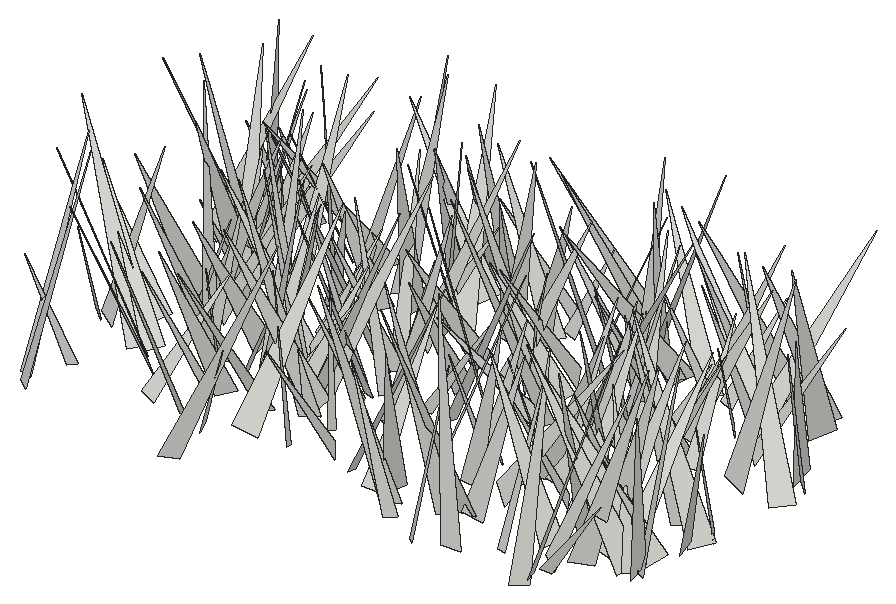
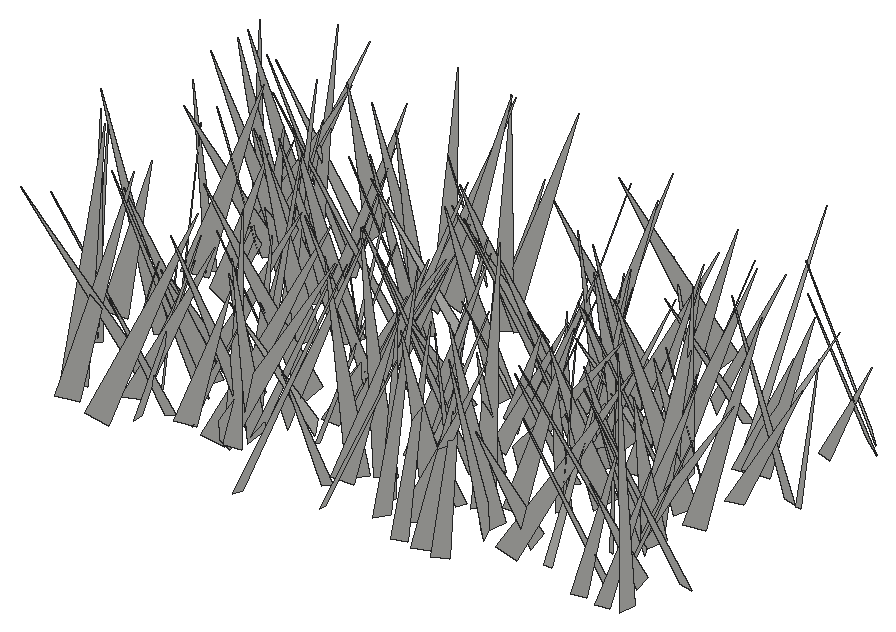
# SketchUp Ruby script. Lengths in inches.
U = 1.inch
M = Sketchup.active_model
def pt(a) = Geom::Point3d.new(a.map { |v| v * U })
def face(e, loops, mat)
  f = e.add_face(loops[0].map { |a| pt(a) })
  loops[1..].each { |l| e.add_face(l.map { |a| pt(a) }).erase! }
  f.material = f.back_material = mat if mat
  f
end
# faces: each face lists its corners as indices into pts; further lists are holes
def faces(e, pts, list, mat = nil) = list.each { |f| face(e, (f[0].is_a?(Array) ? f : [f]).map { |l| l.map { |i| pts[i] } }, mat) }
# xy, xz, yz: faces in a plane at the given z, y or x. An outline is a flat list of corners, or four numbers for a rectangle; further outlines are holes
def ring(l) = l.size == 4 ? [[l[0], l[1]], [l[2], l[1]], [l[2], l[3]], [l[0], l[3]]] : l.each_slice(2).to_a
def flat(e, list, mat, &to3) = list.each { |f| face(e, (f[0].is_a?(Array) ? f : [f]).map { |l| ring(l).map { |u, v| to3.(u, v) } }, mat) }
def xy(e, z, list, mat = nil) = flat(e, list, mat) { |x, y| [x, y, z] }
def xz(e, y, list, mat = nil) = flat(e, list, mat) { |x, z| [x, y, z] }
def yz(e, x, list, mat = nil) = flat(e, list, mat) { |y, z| [x, y, z] }
def lines(e, pts, list) = list.each { |a, b| e.add_line(pt(pts[a]), pt(pts[b])) }
# prism: a flat outline (further loops are holes) pulled along v
def prism(e, loops, v, mat = nil)
  f = face(e, loops, mat); d = Geom::Vector3d.new(v.map { |x| x * U })
  f.pushpull(f.normal.samedirection?(d) ? d.length : -d.length)
end
def box(e, o, s, mat = nil) = prism(e, [[o, [o[0] + s[0], o[1], o[2]], [o[0] + s[0], o[1] + s[1], o[2]], [o[0], o[1] + s[1], o[2]]]], [0, 0, s[2]], mat)
def at(x, y, z, deg = 0) = Geom::Transformation.translation(pt([x, y, z])) * Geom::Transformation.rotation(ORIGIN, Z_AXIS, deg.degrees)
def axes(o, x, y, z) = Geom::Transformation.new([*x, 0, *y, 0, *z, 0, *pt(o).to_a, 1])
def part(name) = M.definitions.add(name)
# library, detail: a bought-in or finely detailed component or shape, given as its bounding box
def library(name, o, s) = part(name).tap { |d| box(d.entities, o, s) }
def detail(e, o, s) = box(e.add_group.entities, o, s)
def put(e, d, t, mat = nil) = e.add_instance(d, t).tap { |i| i.material = mat if mat }
def group(e, t, mat = nil) = e.add_group.tap { |g| g.transformation = t; g.material = mat if mat }.entities
root = M.entities
c1 = part("fur_instance\#9")
p = [[0.8125,0,1.79],[0.67,-0.02,1.48],[0,-0.11,0],[0,0.11,0]]
faces(c1.entities,p,[[0,1,2,3]])
put(root,c1,axes([530.97,285.85,-21.66],[-1.13244,4.66111,1.93868],[4.91983,0.57378,1.4943],[-1.13125,-2.17064,4.55801]))
put(root,c1,axes([515.75,283.15,-21.66],[7.47799,-1.52657,1.95795],[-2.25093,-6.79047,3.30259],[-1.04752,3.69369,6.88067]))
put(root,c1,axes([529.06,288.6,-21.66],[6.38115,-3.67921,0.2036],[-3.55943,-6.25987,-1.56256],[-0.95316,-1.25481,7.1982]))
put(root,c1,axes([536.32,285.05,-21.66],[0.66704,7.88186,2.68055],[8.14998,-1.16705,1.40349],[-1.69907,-2.50365,7.78452]))
put(root,c1,axes([529.87,287.22,-21.66],[-0.48012,-7.554,2.16495],[-7.6037,-0.10085,-2.03814],[-1.98335,2.21526,7.28968]))
put(root,c1,axes([533.84,284.27,-21.66],[3.8094,4.08661,1.06154],[3.80016,-3.94157,1.53675],[-1.84012,0.32005,5.37125]))
put(root,c1,axes([515.07,287.34,-21.66],[4.19489,0.81761,0.41517],[0.91291,-3.90671,-1.53042],[-0.08632,-1.58339,3.99042]))
put(root,c1,axes([542.66,286.41,-21.66],[2.65844,-2.5721,0.0216],[-2.2994,-2.3625,1.67773],[1.15278,1.21916,3.2967]))
put(root,c1,axes([523.16,290.16,-21.66],[-4.76497,-3.93422,0.44703],[-3.2824,4.31602,2.99679],[2.21445,-2.06803,5.40391]))
put(root,c1,axes([542.42,284.16,-21.66],[-6.84761,2.51212,1.52779],[1.98246,6.80446,-2.30302],[2.17135,1.70976,6.92074]))
put(root,c1,axes([534.45,288.99,-21.66],[-1.86183,-7.54983,1.10161],[-7.50699,1.61006,-1.65309],[-1.3633,1.44488,7.59827]))
put(root,c1,axes([503.11,284.7,-21.66],[5.00071,5.94343,0.88428],[5.7504,-5.06729,1.53914],[-1.74336,0.3341,7.61331]))
put(root,c1,axes([533.54,288.07,-21.66],[-0.98581,-7.65367,2.64082],[-7.9173,0.35473,-1.92744],[-1.69382,2.79641,7.47232]))
put(root,c1,axes([513.05,287.875,-21.66],[-3.40667,-4.88664,0.79026],[-4.79108,3.01371,-2.01797],[-1.2447,1.77411,5.60468]))
put(root,c1,axes([507.74,291.31,-21.66],[-4.53794,-6.8341,0.16977],[-6.57814,4.42074,2.12406],[1.86058,-1.03861,7.92377]))
put(root,c1,axes([547.21,289.82,-21.66],[7.02659,-0.33713,1.59],[0.09653,-6.95626,-1.90152],[-1.62247,-1.87389,6.7728]))
put(root,c1,axes([542.24,287.38,-21.66],[3.65176,6.04586,1.11201],[6.02251,-3.25936,-2.05677],[1.23222,-1.98709,6.75703]))
put(root,c1,axes([503.86,288.52,-21.66],[-0.24742,-3.68689,1.2628],[-3.55064,-0.30834,-1.59591],[-1.60648,1.24932,3.33279]))
put(root,c1,axes([542.32,285.37,-21.66],[7.12213,3.78972,1.00867],[3.4176,-7.02352,2.25704],[-1.92338,1.55314,7.74548]))
put(root,c1,axes([546.34,289.97,-21.66],[-7.92246,2.32052,1.49756],[2.68865,7.5204,2.57051],[0.63138,-2.90715,7.84491]))
put(root,c1,axes([542.16,291.02,-21.66],[-1.3783,-7.92591,0.91068],[-7.76861,1.54372,1.6777],[1.81604,0.58822,7.86798]))
put(root,c1,axes([512.99,290.77,-21.66],[-4.86193,-2.9811,0.43497],[-2.74592,4.72474,1.68858],[1.2394,-1.22654,5.44739]))
put(root,c1,axes([540.83,289.375,-21.66],[-5.87282,3.13064,1.60123],[3.47052,5.66214,1.65846],[0.56601,-2.23474,6.44519]))
put(root,c1,axes([513.48,291.58,-21.66],[3.27903,-5.74844,0.73311],[-5.41958,-3.34021,-1.9507],[-2.05188,-0.36394,6.32387]))
put(root,c1,axes([534.95,288.9,-21.66],[-0.35143,6.05342,2.99786],[6.31844,1.35633,-1.99808],[2.38924,-2.69649,5.72495]))
put(root,c1,axes([543.76,288.49,-21.66],[6.10397,-4.61293,1.81963],[-4.95361,-5.80478,1.9013],[-0.22786,2.62185,7.41098]))
put(root,c1,axes([502.4,285.78,-21.66],[3.79972,6.90357,0.39781],[6.61789,-3.76205,2.07507],[-2.00527,0.66563,7.60206]))
put(root,c1,axes([516.72,291.52,-21.66],[0.00181,-5.98408,0.19016],[-5.68264,-0.06159,-1.88392],[-1.88493,0.17992,5.67979]))
put(root,c1,axes([538.9,286.78,-21.66],[2.7978,5.22834,0.27095],[4.99402,-2.75746,1.64099],[-1.57121,0.54549,5.69828]))
put(root,c1,axes([547.18,291.66,-21.66],[-6.27712,3.42033,1.55819],[3.73626,5.34865,3.31076],[-0.40863,-3.63622,6.33559]))
put(root,c1,axes([510.05,288.2,-21.66],[1.05381,5.0713,0.10966],[4.76326,-0.95083,-1.80217],[1.74396,-0.4674,4.856]))
put(root,c1,axes([527.99,287.75,-21.66],[-2.51338,5.74575,1.01303],[5.46798,2.70448,-1.77311],[2.03497,-0.17044,6.01555]))
put(root,c1,axes([520.58,288.82,-21.66],[-5.03149,-1.83162,1.20846],[-2.18082,4.50919,-2.24552],[0.24343,2.5384,4.86091]))
put(root,c1,axes([519.12,293.67,-21.66],[-7.73279,0.49202,2.83462],[1.75633,7.24586,3.53356],[2.27869,-3.91518,6.89581]))
put(root,c1,axes([546.6875,292.45,-21.66],[-4.22388,-0.55824,1.0602],[-0.01996,3.91714,1.98304],[1.19803,-1.90295,3.77099]))
put(root,c1,axes([543.84,290.95,-21.66],[4.37755,-6.1842,1.75356],[-6.40379,-4.01166,1.83857],[0.55746,2.47882,7.3503]))
put(root,c1,axes([546.74,289.47,-21.66],[-0.83276,5.81039,0.96307],[5.68734,0.54058,1.65638],[-1.53047,-1.15272,5.63121]))
put(root,c1,axes([532.32,292.05,-21.66],[1.87666,-6.19619,1.68038],[-6.32701,-1.4881,1.57887],[1.08876,2.03251,6.27868]))
put(root,c1,axes([517.32,288.61,-21.66],[-1.94232,7.80928,1.11049],[7.41359,2.19794,-2.48968],[2.69386,-0.41817,7.65238]))
put(root,c1,axes([525.49,288.91,-21.66],[6.20269,2.14266,0.41588],[1.88774,-5.89525,2.21806],[-1.09562,1.97291,6.17613]))
put(root,c1,axes([538.27,294.13,-21.66],[-4.62318,-3.47557,0.41553],[-3.19467,4.47097,1.85217],[1.4305,-1.24775,5.47931]))
put(root,c1,axes([544.24,290.26,-21.66],[-0.17327,7.80384,1.95788],[7.72096,0.71202,-2.15474],[2.26272,-1.83203,7.50246]))
put(root,c1,axes([519.29,292.49,-21.66],[-0.93338,-7.69941,2.7531],[-7.87622,0.10215,-2.38461],[-2.19672,2.90522,7.38009]))
put(root,c1,axes([547.47,289.7,-21.66],[3.93388,5.26717,1.14139],[4.90502,-4.08461,1.94372],[-2.23307,0.30691,6.28017]))
put(root,c1,axes([542.2,294.74,-21.66],[-5.45284,-1.57742,1.94379],[-0.6971,5.43147,2.45217],[2.40429,-2.00271,5.11943]))
put(root,c1,axes([506.74,292.28,-21.66],[-5.49378,-4.48735,0.1731],[-4.21573,5.05933,-2.64174],[-1.54724,2.14821,6.58325]))
put(root,c1,axes([547.57,293.93,-21.66],[5.98567,0.36805,0.66862],[0.55714,-5.71998,-1.83907],[-0.52163,-1.88604,5.70802]))
put(root,c1,axes([534.47,292.25,-21.66],[4.68753,6.76488,0.69054],[6.04009,-3.75687,-4.19721],[3.12373,-2.88717,7.07954]))
put(root,c1,axes([510.81,294.57,-21.66],[0.32689,-6.93131,1.01824],[-6.72809,-0.59471,-1.88835],[-1.95261,0.88881,6.67713]))
put(root,c1,axes([501.14,294.5,-21.66],[-2.16154,-4.08693,0.6496],[-3.73051,2.24163,1.68984],[1.79115,-0.26331,4.30345]))
put(root,c1,axes([510.66,294.32,-21.66],[-2.98653,-2.99705,1.42564],[-2.58075,3.30304,1.53746],[2.08674,-0.20437,3.94181]))
put(root,c1,axes([532.27,292.78,-21.66],[0.67083,5.9533,2.27987],[6.17356,-0.03505,-1.72498],[1.58958,-2.37626,5.73727]))
put(root,c1,axes([545.71,290.08,-21.66],[-2.00066,7.03095,0.19663],[6.73059,1.97306,-2.06922],[2.04255,0.38513,7.01108]))
put(root,c1,axes([521.4,292.02,-21.66],[-4.31752,-0.25034,0.73123],[-0.52227,4.00392,-1.71296],[0.56974,1.77322,3.97108]))
put(root,c1,axes([539.76,296.52,-21.66],[-3.16207,-7.07316,1.24758],[-6.76016,3.39142,2.09364],[2.42619,0.2311,7.45956]))
put(root,c1,axes([530.11,291.04,-21.66],[5.9455,4.2001,0.21568],[4.05072,-5.81939,1.66213],[-1.13095,1.23699,7.08711]))
put(root,c1,axes([515.97,291.76,-21.66],[6.62272,2.03005,2.53711],[1.31072,-6.93962,2.13125],[-2.97322,1.46257,6.59085]))
put(root,c1,axes([520.82,295.73,-21.66],[-4.32918,-1.79601,0.73607],[-1.48596,4.22424,1.56749],[1.24875,-1.19977,4.41706]))
put(root,c1,axes([506.58,293.13,-21.66],[-3.94655,4.7323,0.06828],[4.56087,3.77904,1.70056],[-1.26405,-1.13963,5.92267]))
put(root,c1,axes([505.78,292.89,-21.66],[-4.22364,6.9226,0.63988],[6.72709,3.88063,2.42031],[-1.75445,-1.78585,7.73974]))
put(root,c1,axes([511.64,297.58,-21.66],[6.11084,-2.63091,1.80363],[-1.49433,-5.80472,-3.40432],[-2.81811,-2.62692,5.71618]))
put(root,c1,axes([532.14,294.27,-21.66],[-1.49858,-3.44059,1.04989],[-3.40031,0.98374,-1.62968],[-1.17382,1.54281,3.38047]))
put(root,c1,axes([501.99,294.28,-21.66],[3.4737,5.90005,1.74495],[6.11319,-3.08303,-1.74525],[0.69596,-2.36778,6.62052]))
put(root,c1,axes([548,296.24,-21.66],[-3.52584,-3.38703,1.52089],[-2.9555,3.82986,1.67745],[2.24724,-0.27722,4.59235]))
put(root,c1,axes([548.17,294.86,-21.66],[-5.06971,5.94983,1.91077],[6.22333,4.58369,2.23904],[-0.56711,-2.88838,7.48926]))
put(root,c1,axes([535.36,295.38,-21.66],[5.33015,-4.46349,0.382],[-4.4244,-5.15196,1.5366],[0.7024,1.41905,6.78027]))
put(root,c1,axes([534.23,296.93,-21.66],[-3.15103,-4.03715,0.66571],[-3.75697,3.18756,1.54769],[1.62077,-0.46003,4.88182]))
put(root,c1,axes([540,293,-21.66],[-2.57926,6.41675,1.59968],[6.21683,2.93816,-1.76197],[2.25493,-0.76079,6.68751]))
put(root,c1,axes([515.35,292.8,-21.66],[-5.11664,3.91829,0.85035],[3.38571,4.96082,-2.48663],[2.14782,1.51438,5.94556]))
put(root,c1,axes([517.5,294.375,-21.66],[-6.96753,-1.64469,0.65915],[-1.76863,6.61713,-2.18437],[0.10697,2.27915,6.81763]))
put(root,c1,axes([532.0625,295.33,-21.66],[-6.33694,-5.31771,1.42218],[-5.44687,5.74429,-2.79146],[-0.79519,3.03026,7.78734]))
put(root,c1,axes([520.47,296.82,-21.66],[-3.35511,-5.27651,0.83113],[-5.27558,3.11951,-1.49198],[-0.83701,1.48869,6.07225]))
put(root,c1,axes([536.2,295.35,-21.66],[0.74046,6.81709,2.01452],[6.9144,-0.22063,-1.79488],[1.64984,-2.13492,6.61811]))
put(root,c1,axes([513.3125,297.99,-21.66],[7.4678,0.08394,0.57516],[0.2355,-7.21321,-2.00499],[-0.53141,-2.01703,7.1941]))
put(root,c1,axes([515.43,296.5625,-21.66],[2.92691,3.10527,0.26779],[2.82947,-2.4932,-2.01476],[1.3071,-1.55642,3.76168]))
put(root,c1,axes([504.56,296.51,-21.66],[-4.43376,3.47486,0.22998],[3.34427,4.14468,1.85019],[-0.97128,-1.59146,5.32068]))
put(root,c1,axes([545.39,296.04,-21.66],[-0.37721,6.24874,2.25952],[6.16262,-0.51732,2.45945],[-2.4848,-2.23161,5.75674]))
put(root,c1,axes([516.48,295.58,-21.66],[0.2906,4.64928,0.9365],[4.41539,0.07727,-1.75374],[1.73123,-0.9775,4.31562]))
put(root,c1,axes([506.51,296.91,-21.66],[3.8282,2.91024,0.83789],[3.01788,-3.55309,-1.44728],[0.25298,-1.65308,4.58585]))
put(root,c1,axes([509.3125,295.1,-21.66],[4.39596,-0.31282,2.17467],[-1.10489,-4.51925,1.5834],[-1.89902,1.90528,4.11281]))
put(root,c1,axes([517.9,294.95,-21.66],[6.72656,-0.08852,1.07497],[-0.40385,-6.50233,1.99163],[-1.00015,2.03024,6.42556]))
put(root,c1,axes([523.47,295.33,-21.66],[6.60662,-2.19065,2.41659],[-2.83754,-6.55209,1.81792],[-1.6085,2.56075,6.71874]))
put(root,c1,axes([512.93,294.11,-21.66],[4.98815,3.01806,0.37753],[2.59556,-4.60182,2.49383],[-1.58564,1.9615,5.26983]))
put(root,c1,axes([515.75,296.23,-21.66],[-7.81157,-0.92448,1.21309],[-1.13809,7.74743,-1.42443],[1.01538,1.5715,7.73604]))
put(root,c1,axes([537.4,297.05,-21.66],[3.87683,-5.48097,2.21285],[-5.90731,-3.50163,1.67625],[0.20355,2.76859,6.50085]))
put(root,c1,axes([523.26,294.76,-21.66],[3.56764,3.88458,0.34534],[3.52617,-3.41301,1.96335],[-1.66594,1.09483,4.89523]))
put(root,c1,axes([514.37,298.71,-21.66],[-6.85321,0.30824,0.48855],[0.41589,6.6696,1.62593],[0.40091,-1.64973,6.66467]))
put(root,c1,axes([504.55,300.46,-21.66],[4.75153,-4.99406,0.9078],[-4.47168,-4.70683,-2.48828],[-2.40183,-1.11663,6.42854]))
put(root,c1,axes([518.02,295.52,-21.66],[3.14457,7.68443,0.45621],[7.56933,-2.99688,-1.69436],[1.40136,-1.05601,8.12822]))
put(root,c1,axes([508.48,296.33,-21.66],[-8.04005,-0.21045,2.18635],[-0.63833,8.16213,-1.56173],[2.10165,1.67397,7.88972]))
put(root,c1,axes([530.3,300.95,-21.66],[-5.57045,-1.42182,0.3414],[-1.0257,4.7578,3.07884],[1.04215,-2.91715,4.85512]))
put(root,c1,axes([524.47,301.14,-21.66],[5.34512,-3.23236,0.64666],[-2.65449,-4.95104,-2.80671],[-1.95449,-2.11559,5.5804]))
put(root,c1,axes([519.36,297.63,-21.66],[-6.43064,-2.17008,0.24743],[-2.17262,6.27662,-1.4168],[-0.22404,1.42068,6.6374]))
put(root,c1,axes([513.97,295.28,-21.66],[-7.73799,2.57835,1.8542],[1.9672,7.72518,-2.53263],[2.4932,1.90688,7.75308]))
put(root,c1,axes([524.48,297.43,-21.66],[3.53802,-1.77872,0.68161],[-1.86523,-2.94336,2.00089],[0.38644,2.07817,3.41729]))
put(root,c1,axes([514.57,298.73,-21.66],[0.74077,3.76285,1.03817],[3.63302,-0.27816,-1.5841],[1.42759,-1.24465,3.49262]))
put(root,c1,axes([520,300.34,-21.66],[0.21984,-5.04241,1.33274],[-4.72838,-0.75562,-2.0789],[-2.20101,1.11963,4.59917]))
put(root,c1,axes([526.34,297.48,-21.66],[6.82155,0.82248,0.97272],[0.53436,-6.65794,1.88216],[-1.15634,1.77527,6.60814]))
put(root,c1,axes([521.23,297.55,-21.66],[0.1109,6.16383,0.84068],[5.38265,-0.51661,3.07768],[-3.11876,-0.67243,5.34163]))
put(root,c1,axes([506.21,299.14,-21.66],[6.24865,-3.61776,1.18124],[-3.80474,-5.99015,1.78079],[-0.08657,2.13519,6.99733]))
put(root,c1,axes([507.19,298.94,-21.66],[4.17015,5.48726,0.52169],[5.30168,-3.81404,-2.26221],[1.50809,-1.76505,6.51019]))
put(root,c1,axes([506.85,302.11,-21.66],[-4.18199,-2.55213,0.91155],[-1.98836,4.02848,2.15666],[1.84139,-1.44616,4.39901]))
put(root,c1,axes([536.92,302.16,-21.66],[-3.51133,-6.12863,1.17286],[-5.90116,3.69891,1.66117],[2.0278,0.152,6.86513]))
put(root,c1,axes([505.61,303.55,-21.66],[5.60712,-6.07402,0.33398],[-5.83929,-5.5015,-2.02021],[-1.70529,-1.13347,8.01575]))
put(root,c1,axes([523.48,304.34,-21.66],[5.96418,-2.86813,1.57613],[-1.66285,-5.47776,-3.67572],[-2.81874,-2.83722,5.50334]))
put(root,c1,axes([518.46,300.56,-21.66],[-5.00631,-5.98003,0.73957],[-5.22244,3.82659,-4.41068],[-3.00563,3.31169,6.43193]))
put(root,c1,axes([531.37,300.82,-21.66],[-3.36679,-6.63148,1.92496],[-6.20382,1.96447,-4.08298],[-3.03226,3.34389,6.21619]))
put(root,c1,axes([540.28,303.22,-21.66],[-1.24481,-6.10899,0.55091],[-5.80958,0.99391,-2.10566],[-1.96776,0.93016,5.86818]))
put(root,c1,axes([513.62,300.85,-21.66],[-0.24087,4.17753,0.95098],[3.88217,0.61574,-1.72155],[1.81241,-0.76371,3.81393]))
put(root,c1,axes([535.84,300.3,-21.66],[2.63979,2.66437,0.28601],[2.37928,-2.51517,1.47039],[-1.23275,0.85099,3.4504]))
put(root,c1,axes([548.02,304.77,-21.66],[-3.37811,-5.89928,1.5704],[-5.1932,3.72048,2.80499],[3.2091,-0.18922,6.19235]))
put(root,c1,axes([544.89,302.07,-21.66],[-0.81294,-7.33898,4.00432],[-7.82592,2.08335,2.22952],[2.94113,3.51498,7.03923]))
put(root,c1,axes([511.96,303.94,-21.66],[0.90872,-5.0896,0.45336],[-4.90772,-0.74115,1.51668],[1.42262,0.69427,4.94262]))
put(root,c1,axes([529.14,306.54,-21.66],[-5.60645,-3.595,0.79099],[-2.74257,5.04084,3.47133],[2.4552,-2.57833,5.68385]))
put(root,c1,axes([547.64,305.26,-21.66],[7.1612,-0.61813,1.17268],[-0.1707,-6.81898,-2.55193],[-1.31459,-2.48182,6.71956]))
put(root,c1,axes([527.31,303.46,-21.66],[3.73633,3.15118,1.53756],[3.50493,-3.41917,-1.50964],[-0.09758,-2.15258,4.64878]))
put(root,c1,axes([530.17,304.08,-21.66],[-4.08347,2.98679,1.40676],[3.27171,3.36098,2.36101],[-0.44252,-2.71247,4.47451]))
put(root,c1,axes([506.64,301.39,-21.66],[-4.46885,1.59045,1.08144],[1.18804,4.43404,-1.61169],[1.51249,1.21632,4.46123]))
put(root,c1,axes([535.125,305.29,-21.66],[4.67947,-2.49587,0.44393],[-2.29207,-4.56374,-1.49753],[-1.08298,-1.12554,5.08765]))
put(root,c1,axes([526.33,303.01,-21.66],[1.93796,6.92662,2.2466],[6.80944,-0.90011,-3.09877],[2.58009,-2.82714,6.49087]))
put(root,c1,axes([533.09,302.04,-21.66],[7.82793,-0.68601,0.13891],[-0.69946,-7.6099,1.83483],[0.02566,1.8399,7.64072]))
put(root,c1,axes([548.9,301.79,-21.66],[-3.56857,7.17935,0.49748],[7.02506,3.35468,1.97986],[-1.56176,-1.31463,7.76903]))
put(root,c1,axes([514.4375,305.74,-21.66],[2.95346,-5.37759,1.21149],[-5.08452,-3.18852,-1.75785],[-2.12927,0.1548,5.87804]))
put(root,c1,axes([538,303.46,-21.66],[1.07989,-3.22676,1.49499],[-3.22529,-0.23045,1.83235],[1.49815,1.82977,2.86716]))
put(root,c1,axes([528.29,304.05,-21.66],[-0.67807,6.71445,3.30984],[6.96597,-0.65101,2.74773],[-2.74118,-3.31527,6.16389]))
put(root,c1,axes([536.34,301.12,-21.66],[4.01654,5.38759,0.39242],[5.219,-3.99648,1.45013],[-1.3936,0.56102,6.56169]))
put(root,c1,axes([516.14,306.63,-21.66],[7.64117,-3.1953,0.94942],[-2.87226,-7.51641,-2.18001],[-1.69158,-1.67105,7.9903]))
put(root,c1,axes([539.35,302.6,-21.66],[3.96425,-0.56902,0.64503],[-0.79665,-3.57598,1.74151],[-0.32433,1.82859,3.60641]))
put(root,c1,axes([522.51,304.13,-21.66],[-5.08452,-4.09315,0.88657],[-4.17476,4.84247,-1.58557],[-0.33349,1.78573,6.33184]))
put(root,c1,axes([506.54,306.03,-21.66],[-2.8265,-4.26887,1.57231],[-3.66111,3.23328,2.19698],[2.70032,-0.08465,4.62446]))
put(root,c1,axes([506.38,303.75,-21.66],[-3.06653,-6.21678,2.70439],[-6.51984,1.89062,-3.04678],[-1.85842,3.62531,6.22648]))
put(root,c1,axes([506.16,303.54,-21.66],[-3.15581,4.82371,2.67558],[4.59437,4.00448,-1.80054],[3.05265,-1.04019,5.47589]))
put(root,c1,axes([518.74,301.99,-21.66],[0.42359,6.38348,0.10104],[6.1795,-0.43539,1.60081],[-1.60398,0.00839,6.194]))
put(root,c1,axes([541.57,301.97,-21.66],[-3.94545,3.07895,0.18102],[2.74281,3.63702,-2.08047],[1.41057,1.53994,4.55172]))
put(root,c1,axes([510.56,301.58,-21.66],[-6.29891,4.40553,1.36932],[3.82289,6.28157,-2.62437],[2.58248,1.44677,7.22479]))
put(root,c1,axes([504.68,306.43,-21.66],[-4.29176,-1.39668,0.34406],[-1.22552,4.11722,1.42648],[0.75311,-1.25938,4.28195]))
put(root,c1,axes([505.99,305.02,-21.66],[-4.67528,-5.85921,0.505],[-5.43274,4.05599,-3.23694],[-2.25181,2.37953,6.76097]))
put(root,c1,axes([518.97,303.89,-21.66],[3.76818,7.24013,0.96766],[7.17608,-3.46602,-2.01138],[1.36373,-1.76699,7.91031]))
put(root,c1,axes([538.77,304.76,-21.66],[3.61026,-5.57217,1.81458],[-5.57053,-2.60139,3.09478],[1.81959,3.09184,5.87413]))
put(root,c1,axes([532.58,305.55,-21.66],[-5.1387,-6.17044,1.38685],[-6.22365,4.61615,-2.52214],[-1.12419,2.64967,7.62361]))
put(root,c1,axes([540.75,307.28,-21.66],[-2.708,-3.38854,1.07596],[-2.8715,2.88211,1.84961],[2.09627,-0.42942,3.92357]))
put(root,c1,axes([523.2,307.3,-21.66],[1.45469,-7.67033,1.86376],[-7.74266,-1.0178,1.85445],[1.53584,2.13396,7.5836]))
put(root,c1,axes([504.99,303.72,-21.66],[-6.13848,3.83375,0.83292],[3.60337,6.1212,-1.61832],[1.55148,0.95163,7.05405]))
put(root,c1,axes([543.63,305.49,-21.66],[3.84668,4.92623,0.09388],[4.62666,-3.57049,-2.21792],[1.69428,-1.43435,5.84342]))
put(root,c1,axes([510.96,305.375,-21.66],[-6.29577,-3.22015,2.48262],[-3.79064,6.30377,-1.43636],[1.47099,2.46225,6.92409]))
put(root,c1,axes([532.69,308.14,-21.66],[-6.28485,-0.79991,0.77187],[-0.56549,6.11624,1.73401],[0.95701,-1.63912,6.09364]))
put(root,c1,axes([534.32,310.37,-21.66],[4.16443,-6.48584,0.7003],[-5.50995,-3.94185,-3.74183],[-3.49241,-1.51483,6.7385]))
put(root,c1,axes([505.3,304.13,-21.66],[5.32876,3.34285,1.26399],[2.90072,-5.37113,1.97605],[-2.08763,1.0697,5.97207]))
put(root,c1,axes([508.51,309.8,-21.66],[-3.43446,-5.67079,0.15135],[-5.3482,3.29577,2.1239],[1.89143,-0.97791,6.28032]))
put(root,c1,axes([535.67,304.44,-21.66],[-5.09281,3.29268,0.78292],[3.01884,5.05892,-1.63872],[1.53013,0.9783,5.83893]))
put(root,c1,axes([511.47,310.18,-21.66],[2.28844,-6.77562,0.58153],[-5.77223,-2.2597,-3.61376],[-3.59563,-0.68473,6.17144]))
put(root,c1,axes([519.42,305.57,-21.66],[-5.36603,-1.88935,2.74168],[-2.67241,5.54565,-1.40882],[1.98613,2.35731,5.51173]))
put(root,c1,axes([524.52,308.35,-21.66],[2.49015,-6.48815,0.76577],[-6.33726,-2.19962,1.97082],[1.58797,1.39602,6.66429]))
put(root,c1,axes([538.21,306.42,-21.66],[4.07945,6.65627,1.20942],[6.56454,-3.55321,-2.58689],[1.63565,-2.3408,7.36585]))
put(root,c1,axes([517.45,307.15,-21.66],[1.13497,4.33314,1.68645],[4.04549,-0.06445,-2.557],[2.29221,-2.03177,3.67778]))
put(root,c1,axes([545.28,310.29,-21.66],[6.81384,-4.6319,0.82302],[-4.34734,-6.75311,-2.01405],[-1.7979,-1.22528,7.98915]))
put(root,c1,axes([521.33,309.4,-21.66],[5.7747,-1.11479,0.95698],[-0.77258,-5.60537,-1.86777],[-1.24967,-1.68603,5.57685]))
put(root,c1,axes([541.55,308.35,-21.66],[-0.61117,-4.98438,1.28841],[-4.9544,0.21679,-1.51148],[-1.3993,1.40945,4.78884]))
put(root,c1,axes([530.46,305.08,-21.66],[5.39727,3.08007,0.18691],[2.81936,-5.07536,2.22356],[-1.25418,1.84558,5.80286]))
put(root,c1,axes([503.61,306.84,-21.66],[4.07618,6.66518,0.05677],[6.29765,-3.82934,-2.59208],[2.18344,-1.39809,7.37028]))
put(root,c1,axes([532.86,310.26,-21.66],[-0.95701,-7.3765,1.52863],[-7.35851,1.24531,1.40248],[1.61303,1.30453,7.30491]))
put(root,c1,axes([500.32,306.57,-21.66],[3.27574,7.01328,0.4286],[6.91428,-3.13335,-1.57325],[1.25002,-1.04703,7.57902]))
put(root,c1,axes([533.96,310.08,-21.66],[-0.88156,-7.55851,1.51866],[-6.98391,0.13553,-3.37952],[-3.26533,1.75074,6.81814]))
put(root,c1,axes([543.74,307.49,-21.66],[-5.8174,-1.77979,0.63377],[-1.88895,5.44209,-2.05595],[-0.03436,2.15114,5.72563]))
put(root,c1,axes([544.56,311.85,-21.66],[4.80853,-5.64104,1.01196],[-5.19564,-4.8483,-2.3381],[-2.41883,-0.80002,7.03396]))
put(root,c1,axes([520.33,311.27,-21.66],[7.53052,-1.13144,2.64431],[-0.30654,-7.68469,-2.41514],[-2.85982,-2.15562,7.22191]))
put(root,c1,axes([539.65,311.04,-21.66],[-5.8383,-2.13052,1.19785],[-1.77007,5.82456,1.73238],[1.68547,-1.263,5.96857]))
put(root,c1,axes([525.01,309.33,-21.66],[-3.75455,5.21199,1.89568],[5.51913,3.28609,1.89629],[-0.5456,-2.62523,6.13723]))
put(root,c1,axes([536.98,309.53,-21.66],[-0.30638,-3.92044,1.36874],[-3.76361,-0.31774,-1.75256],[-1.75458,1.36615,3.52026]))
put(root,c1,axes([541.44,309.29,-21.66],[-6.06762,4.08752,0.30456],[4.00596,5.79855,1.98636],[-0.86766,-1.81261,7.04117]))
put(root,c1,axes([514.07,308.16,-21.66],[6.87844,-2.02965,2.77665],[-2.6588,-7.07628,1.41394],[-2.18175,2.22463,7.03088]))
put(root,c1,axes([519.76,306.8,-21.66],[-5.97227,4.9002,0.90124],[4.6479,5.98621,-1.7477],[1.79477,0.80344,7.52499]))
put(root,c1,axes([501.39,310.93,-21.66],[7.9282,0.66664,2.15118],[1.11346,-8.00329,-1.62351],[-1.9576,-1.85234,7.78877]))
put(root,c1,axes([504.76,311.47,-21.66],[3.23703,-3.40023,0.62778],[-3.13183,-3.24768,-1.44163],[-1.46538,-0.57015,4.46784]))
put(root,c1,axes([502.75,311.67,-21.66],[3.29812,-3.00828,0.87507],[-2.53709,-3.30998,-1.81667],[-1.83812,-0.82908,4.07763]))
put(root,c1,axes([542.24,306.89,-21.66],[1.49345,8.09623,0.02611],[7.76227,-1.42429,-2.34489],[2.30146,-0.44999,7.89182]))
put(root,c1,axes([532.88,307.93,-21.66],[7.43701,2.08557,1.03262],[1.85087,-7.39668,1.60887],[-1.41074,1.29018,7.55449]))
put(root,c1,axes([532.56,308.27,-21.66],[-6.83852,1.49302,2.47832],[0.97247,7.17644,-1.63995],[2.72497,1.18576,6.80477]))
put(root,c1,axes([517.67,312.93,-21.66],[-0.91329,-6.82842,0.06821],[-6.63421,0.90353,1.6239],[1.61843,-0.14959,6.69511]))
put(root,c1,axes([502.67,307.89,-21.66],[4.59265,0.40937,1.72839],[-0.43371,-4.3881,2.19176],[-1.72245,2.19644,4.05662]))
put(root,c1,axes([541.54,312.71,-21.66],[1.64942,-7.33453,1.1804],[-6.83961,-1.97125,-2.69132],[-2.89974,0.47759,7.01946]))
put(root,c1,axes([503.59,309.83,-21.66],[3.2036,5.15972,0.63397],[4.7617,-2.61371,-2.78969],[2.08586,-1.95793,5.39475]))
put(root,c1,axes([518.72,310.87,-21.66],[-6.43604,2.78332,0.65453],[2.85741,6.20344,1.71766],[-0.1023,-1.83529,6.79846]))
put(root,c1,axes([538.4,309.45,-21.66],[0.79551,4.29487,0.6755],[4.10301,-0.51451,-1.56067],[1.4379,-0.90797,4.07959]))
put(root,c1,axes([514.33,313.11,-21.66],[6.011,-2.52803,0.45147],[-2.2406,-5.7244,-2.22212],[-1.25478,-1.8887,6.13068]))
put(root,c1,axes([523.875,312.67,-21.66],[-4.91943,-1.92287,0.32626],[-1.70701,4.67316,1.80343],[0.9434,-1.57124,4.96446]))
put(root,c1,axes([525.36,310.35,-21.66],[0.91676,-3.52562,1.5814],[-3.59518,-0.18259,1.67709],[1.41617,1.81877,3.23385]))
put(root,c1,axes([515.92,313.03,-21.66],[4.34994,-4.04005,0.73934],[-3.73736,-4.34022,-1.72779],[-1.70317,-0.79441,5.67968]))
put(root,c1,axes([536.98,309.72,-21.66],[-3.95209,5.35159,0.47213],[5.26841,3.74586,1.6413],[-1.05182,-1.34553,6.44707]))
put(root,c1,axes([510.95,307.8,-21.66],[5.49101,0.89671,2.25711],[-0.37206,-5.20349,2.97239],[-2.40004,2.85822,4.70322]))
put(root,c1,axes([529.14,314.4,-21.66],[-7.53778,-2.79862,0.78068],[-2.32716,7.11502,3.03655],[1.73954,-2.60846,7.44512]))
put(root,c1,axes([514.14,308.65,-21.66],[-6.72177,-1.11045,3.37602],[-2.29516,6.87097,-2.30972],[2.71346,3.06096,6.4094]))
